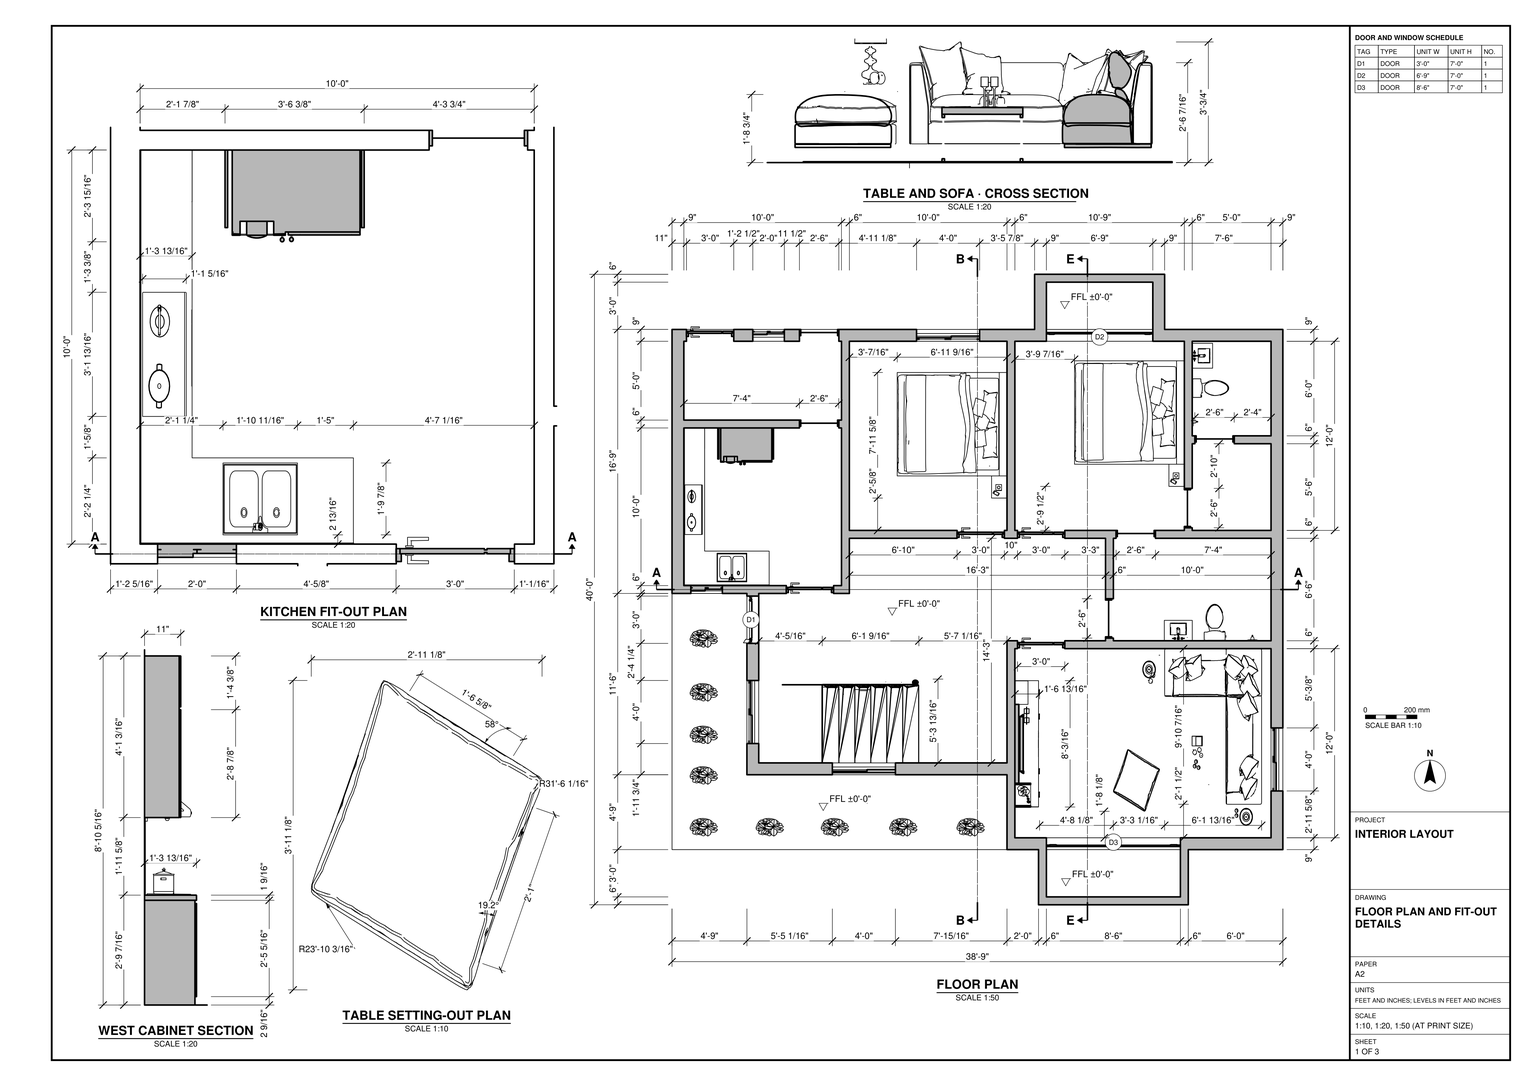
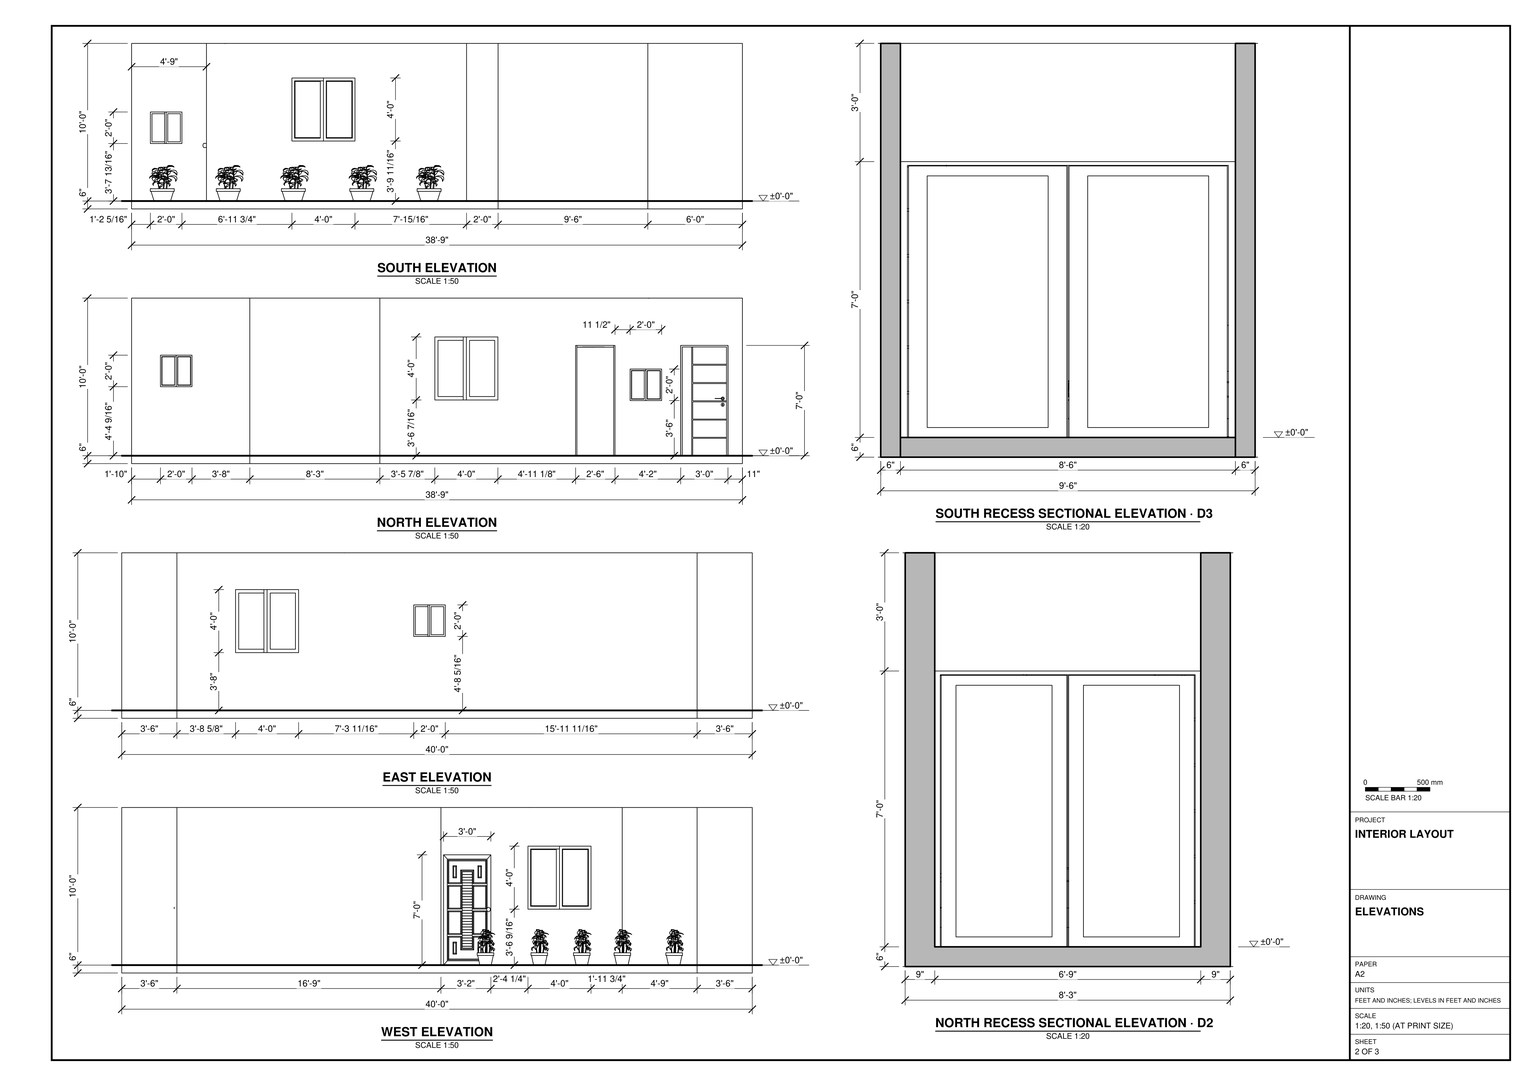
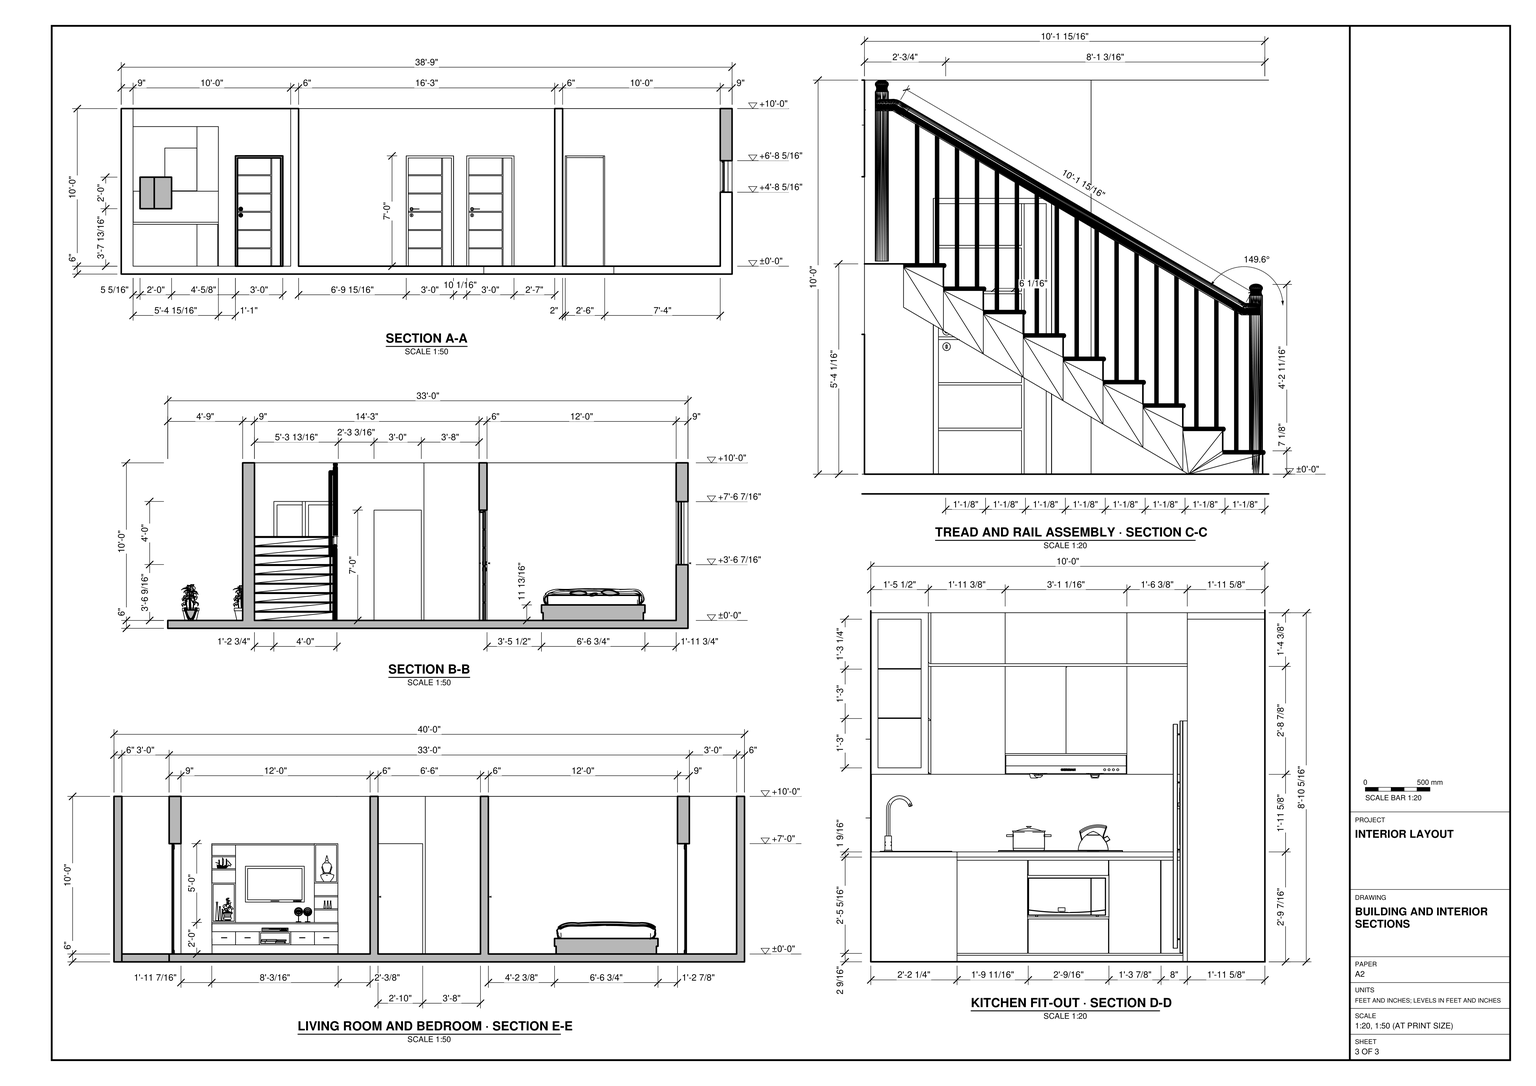
Build the interior in SketchUp using task_files/diagram_01.pdf. Work in feet and inches. Set the finished floor at ±0'-0". The overall model is 38'-9" east to west, 40'-0" north to south and 10'-6" high. Use the floor plan for the stepped perimeter and room positions, the elevations for the openings, and the sections for vertical dimensions.

Model the 6" floor slab, the 10'-0" wall height, and the wall thicknesses shown in plan, including the returns around the north and south recesses. Fit the doors and window units into their openings. Place the kitchen on the west side, the two bedrooms side by side to the north, the bathroom fixtures along the east side and the living room to the southeast. Build the stair off the central circulation space with individual treads, posts, balusters and a sloping handrail.

Use the kitchen details to set out the counters, sink, cooktop, base cabinets, wall cabinets and tall end unit. Position the beds as drawn. In the living room, arrange the corner sofa and angled table opposite the built-in media unit. Decor and loose items, including plants, cushions and appliances, may be any suitable library components.

Keep the shell elements and each furniture or joinery piece in separate groups or components, and use components for repeated parts. Save one SketchUp model as output_files/two_bedroom_interior_with_stair_and_fitted_kitchen.skp.

# SketchUp Ruby script. Lengths in inches.
U = 1.inch
M = Sketchup.active_model
def pt(a) = Geom::Point3d.new(a.map { |v| v * U })
def face(e, loops, mat)
  f = e.add_face(loops[0].map { |a| pt(a) })
  loops[1..].each { |l| e.add_face(l.map { |a| pt(a) }).erase! }
  f.material = f.back_material = mat if mat
  f
end
# faces: each face lists its corners as indices into pts; further lists are holes
def faces(e, pts, list, mat = nil) = list.each { |f| face(e, (f[0].is_a?(Array) ? f : [f]).map { |l| l.map { |i| pts[i] } }, mat) }
# xy, xz, yz: faces in a plane at the given z, y or x. An outline is a flat list of corners, or four numbers for a rectangle; further outlines are holes
def ring(l) = l.size == 4 ? [[l[0], l[1]], [l[2], l[1]], [l[2], l[3]], [l[0], l[3]]] : l.each_slice(2).to_a
def flat(e, list, mat, &to3) = list.each { |f| face(e, (f[0].is_a?(Array) ? f : [f]).map { |l| ring(l).map { |u, v| to3.(u, v) } }, mat) }
def xy(e, z, list, mat = nil) = flat(e, list, mat) { |x, y| [x, y, z] }
def xz(e, y, list, mat = nil) = flat(e, list, mat) { |x, z| [x, y, z] }
def yz(e, x, list, mat = nil) = flat(e, list, mat) { |y, z| [x, y, z] }
def lines(e, pts, list) = list.each { |a, b| e.add_line(pt(pts[a]), pt(pts[b])) }
# prism: a flat outline (further loops are holes) pulled along v
def prism(e, loops, v, mat = nil)
  f = face(e, loops, mat); d = Geom::Vector3d.new(v.map { |x| x * U })
  f.pushpull(f.normal.samedirection?(d) ? d.length : -d.length)
end
def box(e, o, s, mat = nil) = prism(e, [[o, [o[0] + s[0], o[1], o[2]], [o[0] + s[0], o[1] + s[1], o[2]], [o[0], o[1] + s[1], o[2]]]], [0, 0, s[2]], mat)
def at(x, y, z, deg = 0) = Geom::Transformation.translation(pt([x, y, z])) * Geom::Transformation.rotation(ORIGIN, Z_AXIS, deg.degrees)
def axes(o, x, y, z) = Geom::Transformation.new([*x, 0, *y, 0, *z, 0, *pt(o).to_a, 1])
def part(name) = M.definitions.add(name)
# library, detail: a bought-in or finely detailed component or shape, given as its bounding box
def library(name, o, s) = part(name).tap { |d| box(d.entities, o, s) }
def detail(e, o, s) = box(e.add_group.entities, o, s)
def put(e, d, t, mat = nil) = e.add_instance(d, t).tap { |i| i.material = mat if mat }
def group(e, t, mat = nil) = e.add_group.tap { |g| g.transformation = t; g.material = mat if mat }.entities
root = M.entities
M.materials.add("Polis06_194").color = [79, 50, 36]
M.materials.add("[0055_LightGoldenrodYellow]").color = [250, 250, 210]
M.materials.add("[Blacktop Old 01]").color = [132, 136, 139]
M.materials.add("[Concrete Tile]").color = [203, 190, 164]
M.materials.add("[Grass Dark Green]").color = [106, 157, 55]
M.materials.add("[Translucent Glass Blue]").color = [100, 149, 237]
M.materials["[Translucent Glass Blue]"].alpha = 0.5
c1 = library("devendra+jangid+[door]+drawings",[57.04,80.03,0],[48,84,6.66])
c2 = part("Janela aluminio")
xy(c2.entities,0,[[0,0,47.24,1.57],[23.62,1.57,47.24,2.76],[0,2.76,25.98,3.9375],[0,3.9375,47.24,5.91]])
xy(c2.entities,43.31,[[0,0,47.24,1.57],[23.62,1.57,47.24,2.76],[0,2.76,0,5.91,47.24,5.91,47.24,3.9375,25.98,3.9375,25.98,2.76],[25.98,2.76,47.24,3.9375]])
xz(c2.entities,1.57,[[0,0,23.62,0,23.62,41.34,21.26,41.34,21.26,1.97,1.97,1.97,1.97,41.34,23.62,41.34,23.62,43.31,0,43.31],[[23.62,0,47.24,43.31],[25.7,1.97,45.28,41.34]]])
xz(c2.entities,2.76,[[[0,0,23.62,43.31],[2.36,2.36,21.26,40.94]],[23.62,0,25.98,43.31]])
xz(c2.entities,2.76,[[2.36,2.36,21.26,40.94]],"[Translucent Glass Blue]")
xz(c2.entities,3.9375,[[25.98,0,25.98,2.36,44.88,2.36,44.88,40.94,25.98,40.94,25.98,43.31,47.24,43.31,47.24,0]])
xz(c2.entities,3.9375,[[25.98,2.36,44.88,40.94]],"[Translucent Glass Blue]")
yz(c2.entities,0,[[0,0,1.57,43.31],[2.76,0,5.91,43.31]])
yz(c2.entities,23.62,[[1.57,0,2.76,43.31]])
yz(c2.entities,25.98,[[2.76,0,3.9375,43.31]])
yz(c2.entities,47.24,[[0,0,1.57,43.31],[1.57,0,2.76,43.31],[3.9375,0,5.91,43.31]])
c3 = library("Glass+Door",[0,0,0],[72,5.22,111.09])
c4 = library("PINTU+6+YA (1)",[0,-0.6875,0],[35.83,8.07,80.71])
c5 = part("Interior door")
xy(c5.entities,0,[[0,0,4.72,1.18],[0,34.25,4.72,35.43]],"Polis06_194")
xy(c5.entities,85.26,[[0,1.18,4.72,34.25]],"Polis06_194")
xy(c5.entities,86.61,[[0,0,4.72,35.43]],"Polis06_194")
xz(c5.entities,0,[[0,0,4.72,86.61]],"Polis06_194")
xz(c5.entities,1.18,[[0,0,2.36,85.26],[2.36,0,4.72,85.26]],"Polis06_194")
xz(c5.entities,34.25,[[0,0,4.72,85.26]],"Polis06_194")
xz(c5.entities,35.43,[[0,0,4.72,86.61]],"Polis06_194")
yz(c5.entities,0,[[0,0,1.18,86.61],[34.25,0,35.43,86.61],[1.18,85.26,34.25,86.61]],"Polis06_194")
yz(c5.entities,2.36,[[1.18,0,34.25,0,34.25,85.21,1.18,85.26]],"Polis06_194")
yz(c5.entities,4.72,[[0,0,1.18,86.61],[34.25,0,35.43,86.61],[1.18,85.26,34.25,86.61]],"Polis06_194")
c6 = library("Double bed",[0,0,0],[83.59,95.6,35.43])
c7 = library("TS396-4",[-0.02,-3.5,-3.5],[8.95,7,28.74])
c8 = library("K-3457 - Kohler Devonshire(R) elongated toilet with left-han",[-8.99,-6.22,0],[17.99,30.87,31.5])
c9 = library("30\" Kohler Jacquard Vanity",[0,0,0],[30,21.875,40.63])
c10 = library("Flower+pot",[-3.29,-4.11,0],[8.25,8.08,16.09])
c11 = library("Group\#2",[-0.25,0,0],[146.68,133.7,46.53])
c12 = library("Group\#38",[0,83.59,1],[18.8125,96.19,84])
c13 = library("Group\#59",[0,0,0],[37.83,27.94,106.3])
c14 = library("Group\#117",[0,0,0],[96.93,107.95,106.3])
c15 = library("Group\#137",[0,0,0],[107.26,64.92,118.05])
xy(root,0,[[279,0,279,42,285,42,285,6,387,6,387,42,393,42,393,0],[285,6,387,42],[0,42,465,438],[276,438,375,480]])
xy(root,6,[[285,6,387,42],[279,42,285,51],[285,42,387,51],[387,42,393,51],[285,429,366,438],
  [285,438,366,474]],"[0055_LightGoldenrodYellow]")
xy(root,6,[[[261,51,456,51,456,195,299,195,299,201,330,201,330,203,336,203,336,201,456,201,456,279,368,279,368,285,390,285,390,287,396,287,396,285,456,285,456,351,428,351,428,357,456,357,456,429,396,429,396,357,398,357,398,351,396,351,396,317,390,317,390,429,261,429,261,285,263,285,263,279,253,279,253,285,255,285,255,429,135,429,135,285,217,285,217,279,135,279,135,237,123,237,123,243,129,243,129,363,127,363,127,369,129,369,129,429,127,429,127,438,97,438,97,429,47,429,47,438,11,438,11,429,9,429,9,369,97,369,97,363,9,363,9,243,87,243,87,237,66,237,66,235,57,235,57,199,66,199,66,108,255,108,255,201,263,201,263,195,261,195],[330,233,330,279,299,279,299,285,338,285,338,279,336,279,336,233]]],"[Concrete Tile]")
xy(root,6,[[0,42,255,42,255,99,57,99,57,237,0,237]],"[Grass Dark Green]")
xy(root,48,[[61.5,429,85.5,438]],"[Blacktop Old 01]")
xy(root,48.44,[[186.15,429,234.15,438]],"[Blacktop Old 01]")
xy(root,48.58,[[57,122.75,66,170.75]],"[Blacktop Old 01]")
xy(root,49.79,[[14.32,237,38.32,243]],"[Blacktop Old 01]")
xy(root,49.99,[[456,86.64,465,134.64]],"[Blacktop Old 01]")
xy(root,51.67,[[122.0625,99,170.0625,108]],"[Blacktop Old 01]")
xy(root,58.57,[[419.02,429,443.02,438]],"[Blacktop Old 01]")
xy(root,62.33,[[456,222.3,465,246.3]],"[Blacktop Old 01]")
xy(root,72,[[61.5,429,85.5,438]],"[Blacktop Old 01]")
xy(root,73.79,[[14.32,237,38.32,243]],"[Blacktop Old 01]")
xy(root,82.57,[[419.02,429,443.02,438]],"[Blacktop Old 01]")
xy(root,86.33,[[456,222.3,465,246.3]],"[Blacktop Old 01]")
xy(root,90,[[285,42,387,51],[57,199,66,235],[11,429,47,438],[97,429,127,438],[285,429,366,438]])
xy(root,90,[[263,195,299,201],[330,203,336,233],[87,237,123,243],[217,279,253,285],[263,279,299,285],
  [338,279,368,285],[390,287,396,317],[398,351,428,357],[97,363,127,369]],"[0055_LightGoldenrodYellow]")
xy(root,96.44,[[186.15,429,234.15,438]],"[Blacktop Old 01]")
xy(root,96.58,[[57,122.75,66,170.75]],"[Blacktop Old 01]")
xy(root,97.99,[[456,86.64,465,134.64]],"[Blacktop Old 01]")
xy(root,99.67,[[122.0625,99,170.0625,108]],"[Blacktop Old 01]")
xy(root,126,[[[279,0,393,0,393,42,465,42,465,438,375,438,375,480,276,480,276,438,0,438,0,237,57,237,57,99,255,99,255,42,279,42],[66,108,66,237,135,237,135,279,330,279,330,201,255,201,255,108],[261,51,456,195],[261,285,390,429],[135,285,255,429],[9,243,129,363],[336,201,456,279],[9,369,129,429],[396,357,456,429],[396,285,456,351],[285,6,387,42],[285,438,366,474]]],"[0055_LightGoldenrodYellow]")
xz(root,0,[[279,0,393,126]],"[Blacktop Old 01]")
xz(root,6,[[285,0,387,6]])
xz(root,6,[[285,6,387,126]],"[0055_LightGoldenrodYellow]")
xz(root,42,[[285,90,387,126]],"[0055_LightGoldenrodYellow]")
xz(root,42,[[0,0,279,0,279,126,255,126,255,6,0,6],[279,0,285,6],[285,0,387,6],[387,0,393,6],[393,0,465,126]],"[Blacktop Old 01]")
xz(root,51,[[261,6,261,126,456,126,456,6,387,6,387,90,285,90,285,6]],"[0055_LightGoldenrodYellow]")
xz(root,86.64,[[456,49.99,465,97.99]],"[Blacktop Old 01]")
xz(root,99,[[[57,6,255,126],[122.0625,51.67,170.0625,99.67]]],"[Blacktop Old 01]")
xz(root,108,[[[66,6,255,126],[122.0625,51.67,170.0625,99.67]]],"[0055_LightGoldenrodYellow]")
xz(root,122.75,[[57,48.58,66,96.58]],"[Blacktop Old 01]")
xz(root,134.64,[[456,49.99,465,97.99]],"[Blacktop Old 01]")
xz(root,170.75,[[57,48.58,66,96.58]],"[Blacktop Old 01]")
xz(root,195,[[261,6,263,6,263,90,299,90,299,6,456,6,456,126,261,126]],"[0055_LightGoldenrodYellow]")
xz(root,199,[[57,6,66,90]],"[0055_LightGoldenrodYellow]")
xz(root,201,[[255,6,255,126,330,126,330,6,299,6,299,90,263,90,263,6],[336,6,456,126]],"[0055_LightGoldenrodYellow]")
xz(root,203,[[330,6,336,90]],"[0055_LightGoldenrodYellow]")
xz(root,222.3,[[456,62.33,465,86.33]],"[Blacktop Old 01]")
xz(root,233,[[330,6,336,90]],"[0055_LightGoldenrodYellow]")
xz(root,235,[[57,6,66,90]],"[0055_LightGoldenrodYellow]")
xz(root,237,[[66,6,87,6,87,90,123,90,123,6,135,6,135,126,66,126]],"[0055_LightGoldenrodYellow]")
xz(root,237,[[[0,6,57,126],[14.32,49.79,38.32,73.79]]],"[Blacktop Old 01]")
xz(root,243,[[[9,6,9,126,129,126,129,6,123,6,123,90,87,90,87,6],[14.32,49.79,38.32,73.79]]],"[0055_LightGoldenrodYellow]")
xz(root,246.3,[[456,62.33,465,86.33]],"[Blacktop Old 01]")
xz(root,279,[[135,6,217,6,217,90,253,90,253,6,263,6,263,90,299,90,299,6,330,6,330,126,135,126],[336,6,338,6,338,90,368,90,368,6,456,6,456,126,336,126]],"[0055_LightGoldenrodYellow]")
xz(root,285,[[135,6,135,126,255,126,255,6,253,6,253,90,217,90,217,6],[261,6,261,126,390,126,390,6,368,6,368,90,338,90,338,6,299,6,299,90,263,90,263,6],[396,6,456,126]],"[0055_LightGoldenrodYellow]")
xz(root,287,[[390,6,396,90]],"[0055_LightGoldenrodYellow]")
xz(root,317,[[390,6,396,90]],"[0055_LightGoldenrodYellow]")
xz(root,351,[[396,6,398,6,398,90,428,90,428,6,456,6,456,126,396,126]],"[0055_LightGoldenrodYellow]")
xz(root,357,[[396,6,396,126,456,126,456,6,428,6,428,90,398,90,398,6]],"[0055_LightGoldenrodYellow]")
xz(root,363,[[9,6,97,6,97,90,127,90,127,6,129,6,129,126,9,126]],"[0055_LightGoldenrodYellow]")
xz(root,369,[[9,6,9,126,129,126,129,6,127,6,127,90,97,90,97,6]],"[0055_LightGoldenrodYellow]")
xz(root,429,[[[9,6,11,6,11,90,47,90,47,6,97,6,97,90,127,90,127,6,129,6,129,126,9,126],[61.5,48,85.5,72]],[[135,6,255,126],[186.15,48.44,234.15,96.44]],[261,6,285,6,285,90,366,90,366,6,390,6,390,126,261,126],[[396,6,456,126],[419.02,58.57,443.02,82.57]]],"[0055_LightGoldenrodYellow]")
xz(root,438,[[285,90,366,126]],"[0055_LightGoldenrodYellow]")
xz(root,438,[[[0,0,276,126],[11,6,47,90],[97,6,127,90],[186.15,48.44,234.15,96.44],[61.5,48,85.5,72]],[[375,0,465,126],[419.02,58.57,443.02,82.57]]],"[Blacktop Old 01]")
xz(root,474,[[285,6,366,126]],"[0055_LightGoldenrodYellow]")
xz(root,480,[[276,0,375,126]],"[Blacktop Old 01]")
yz(root,0,[[42,0,42,6,237,6,237,126,438,126,438,0]],"[Blacktop Old 01]")
yz(root,9,[[243,6,363,126],[369,6,429,126]],"[0055_LightGoldenrodYellow]")
yz(root,11,[[429,6,438,90]],"[0055_LightGoldenrodYellow]")
yz(root,14.32,[[237,49.79,243,73.79]],"[Blacktop Old 01]")
yz(root,38.32,[[237,49.79,243,73.79]],"[Blacktop Old 01]")
yz(root,47,[[429,6,438,90]],"[0055_LightGoldenrodYellow]")
yz(root,57,[[[99,6,99,126,237,126,237,6,235,6,235,90,199,90,199,6],[122.75,48.58,170.75,96.58]]],"[Blacktop Old 01]")
yz(root,61.5,[[429,48,438,72]],"[Blacktop Old 01]")
yz(root,66,[[[108,6,199,6,199,90,235,90,235,6,237,6,237,126,108,126],[122.75,48.58,170.75,96.58]]],"[0055_LightGoldenrodYellow]")
yz(root,85.5,[[429,48,438,72]],"[Blacktop Old 01]")
yz(root,87,[[237,6,243,90]],"[0055_LightGoldenrodYellow]")
yz(root,97,[[363,6,369,90],[429,6,438,90]],"[0055_LightGoldenrodYellow]")
yz(root,122.0625,[[99,51.67,108,99.67]],"[Blacktop Old 01]")
yz(root,123,[[237,6,243,90]],"[0055_LightGoldenrodYellow]")
yz(root,127,[[363,6,369,90],[429,6,438,90]],"[0055_LightGoldenrodYellow]")
yz(root,129,[[243,6,363,126],[369,6,429,126]],"[0055_LightGoldenrodYellow]")
yz(root,135,[[237,6,279,126],[285,6,429,126]],"[0055_LightGoldenrodYellow]")
yz(root,170.0625,[[99,51.67,108,99.67]],"[Blacktop Old 01]")
yz(root,186.15,[[429,48.44,438,96.44]],"[Blacktop Old 01]")
yz(root,217,[[279,6,285,90]],"[0055_LightGoldenrodYellow]")
yz(root,234.15,[[429,48.44,438,96.44]],"[Blacktop Old 01]")
yz(root,253,[[279,6,285,90]],"[0055_LightGoldenrodYellow]")
yz(root,255,[[108,6,201,126],[285,6,429,126]],"[0055_LightGoldenrodYellow]")
yz(root,255,[[42,6,99,126]],"[Blacktop Old 01]")
yz(root,261,[[51,6,195,126],[285,6,429,126]],"[0055_LightGoldenrodYellow]")
yz(root,263,[[195,6,201,90],[279,6,285,90]],"[0055_LightGoldenrodYellow]")
yz(root,276,[[438,0,480,126]],"[Blacktop Old 01]")
yz(root,279,[[0,0,42,126]],"[Blacktop Old 01]")
yz(root,285,[[6,0,42,6]])
yz(root,285,[[6,6,51,6,51,90,42,90,42,126,6,126],[429,6,474,6,474,126,438,126,438,90,429,90]],"[0055_LightGoldenrodYellow]")
yz(root,299,[[195,6,201,90],[279,6,285,90]],"[0055_LightGoldenrodYellow]")
yz(root,330,[[201,6,201,126,279,126,279,6,233,6,233,90,203,90,203,6]],"[0055_LightGoldenrodYellow]")
yz(root,336,[[201,6,203,6,203,90,233,90,233,6,279,6,279,126,201,126]],"[0055_LightGoldenrodYellow]")
yz(root,338,[[279,6,285,90]],"[0055_LightGoldenrodYellow]")
yz(root,366,[[429,6,429,90,438,90,438,126,474,126,474,6]],"[0055_LightGoldenrodYellow]")
yz(root,368,[[279,6,285,90]],"[0055_LightGoldenrodYellow]")
yz(root,375,[[438,0,480,126]],"[Blacktop Old 01]")
yz(root,387,[[6,0,42,6]])
yz(root,387,[[6,6,6,126,42,126,42,90,51,90,51,6]],"[0055_LightGoldenrodYellow]")
yz(root,390,[[285,6,285,126,429,126,429,6,317,6,317,90,287,90,287,6]],"[0055_LightGoldenrodYellow]")
yz(root,393,[[0,0,42,126]],"[Blacktop Old 01]")
yz(root,396,[[285,6,287,6,287,90,317,90,317,6,351,6,351,126,285,126],[357,6,429,126]],"[0055_LightGoldenrodYellow]")
yz(root,398,[[351,6,357,90]],"[0055_LightGoldenrodYellow]")
yz(root,419.02,[[429,58.57,438,82.57]],"[Blacktop Old 01]")
yz(root,428,[[351,6,357,90]],"[0055_LightGoldenrodYellow]")
yz(root,443.02,[[429,58.57,438,82.57]],"[Blacktop Old 01]")
yz(root,456,[[[51,6,195,126],[86.64,49.99,134.64,97.99]],[[201,6,279,126],[222.3,62.33,246.3,86.33]],[285,6,351,126],[357,6,429,126]],"[0055_LightGoldenrodYellow]")
yz(root,465,[[[42,0,438,126],[86.64,49.99,134.64,97.99],[222.3,62.33,246.3,86.33]]],"[Blacktop Old 01]")
p = [[261,51,6],[255,51,6],[129,429,6],[129,438,6]]
lines(root,p,[[0,1],[2,3]])
put(root,c1,axes([66,277.78,-74.03],[0,-0.75,0],[0,0,1],[-1.75021,0,0]))
put(root,c2,axes([122.0625,99,51.67],[1.016,0,0],[0,1,0],[0,0,1.10836]))
put(root,c3,axes([285,429,6],[1.125,0,0],[0,1.27,0],[0,0,0.75611]))
put(root,c4,axes([263,195.6875,6],[1.00475,0,0],[0,1,0],[0,0,1.04078]))
put(root,c5,axes([330,203,6],[1,0,0],[0,0.84667,0],[0,0,0.96982]))
put(root,c4,axes([263,279.6875,6],[1.00475,0,0],[0,1,0],[0,0,1.04078]))
put(root,c4,axes([216.9375,279.6875,6],[1.00475,0,0],[0,1,0],[0,0,1.04078]))
put(root,c4,axes([86.9375,237.6875,6],[1.00475,0,0],[0,1,0],[0,0,1.04078]))
put(root,c5,axes([390,287,6],[1,0,0],[0,0.84667,0],[0,0,0.96982]))
put(root,c5,axes([338,285,6],[0,-1,0],[0.84667,0,0],[0,0,0.96982]))
put(root,c5,axes([398,357,6],[0,-1,0],[0.84667,0,0],[0,0,0.96982]))
put(root,c5,axes([97,369,6],[0,-1,0],[0.84667,0,0],[0,0,0.96982]))
put(root,c5,axes([97,438,6],[0,-1,0],[0.84667,0,0],[0,0,0.96982]))
put(root,c4,axes([10.9375,432.6875,6],[1.00475,0,0],[0,1,0],[0,0,1.04078]))
put(root,c3,axes([387,51,6],[-1.41667,0,0],[0,-1.27,0],[0,0,0.75611]))
put(root,c6,at(306.41,318.52,6))
put(root,c6,at(171.41,309.63,6))
put(root,c7,axes([441.83,201.01,41.49],[0,1,0],[1.1793,0,0],[0,0,1.85]))
put(root,c8,axes([413.07,206.9,6],[0.89,0,0],[0,0.89,0],[0,0,0.89]))
put(root,c9,axes([396.04,216.53,6],[-0.71,0,0],[0,-0.71,0],[0,0,0.71]))
put(root,c8,axes([401.9,393.34,6],[0,-0.7921,0],[0.89,0,0],[0,0,0.89]))
put(root,c9,axes([411.53,408.5,6],[0,0.6319,0],[-0.71,0,0],[0,0,0.71]))
put(root,c7,axes([396.01,367.75,41.49],[1,0,0],[0,-1.04958,0],[0,0,1.85]))
put(root,c2,axes([186.15,429,48.44],[1.016,0,0],[0,1,0],[0,0,1.10836]))
put(root,c2,axes([57,170.75,48.58],[0,-1.016,0],[1,0,0],[0,0,1.10836]))
put(root,c2,axes([456,134.64,49.99],[0,-1.016,0],[1,0,0],[0,0,1.10836]))
put(root,c2,axes([456,246.3,62.33],[0,-0.508,0],[1,0,0],[0,0,0.55418]))
put(root,c2,axes([443.02,438,58.57],[-0.508,0,0],[0,-1,0],[0,0,0.55418]))
put(root,c2,axes([85.5,438,48],[-0.508,0,0],[0,-1,0],[0,0,0.55418]))
put(root,c2,axes([38.32,242.91,49.79],[-0.508,0,0],[0,-1,0],[0,0,0.55418]))
put(root,c10,axes([225.37,58.55,6],[2.89,0,0],[0,2,0],[0,0,1.7]))
put(root,c10,axes([174.12,58.55,6],[2.89,0,0],[0,2,0],[0,0,1.7]))
put(root,c10,axes([122.06,58.55,6],[2.89,0,0],[0,2,0],[0,0,1.7]))
put(root,c10,axes([72.49,58.55,6],[2.89,0,0],[0,2,0],[0,0,1.7]))
put(root,c10,axes([22.24,58.55,6],[2.89,0,0],[0,2,0],[0,0,1.7]))
put(root,c10,axes([22.24,97.99,6],[2.89,0,0],[0,2,0],[0,0,1.7]))
put(root,c10,axes([22.24,128.86,6],[2.89,0,0],[0,2,0],[0,0,1.7]))
put(root,c10,axes([22.24,161.24,6],[2.89,0,0],[0,2,0],[0,0,1.7]))
put(root,c10,axes([22.24,202.17,6],[2.89,0,0],[0,2,0],[0,0,1.7]))
put(root,c11,axes([335.93,51,6],[0.82,0,0],[0,1.07707,0],[0,0,1]))
put(root,c12,at(261,-9.15,5))
put(root,c13,axes([77.23,363,6],[-1.12,0,0],[0,-1,0],[0,0,1]))
put(root,c14,axes([9,243,6],[0.67,0,0],[0,1.11163,0],[0,0,1]))
put(root,c15,axes([66,106.88,6],[1.16,0,0],[0,1,0],[0,0,1.01655]))
